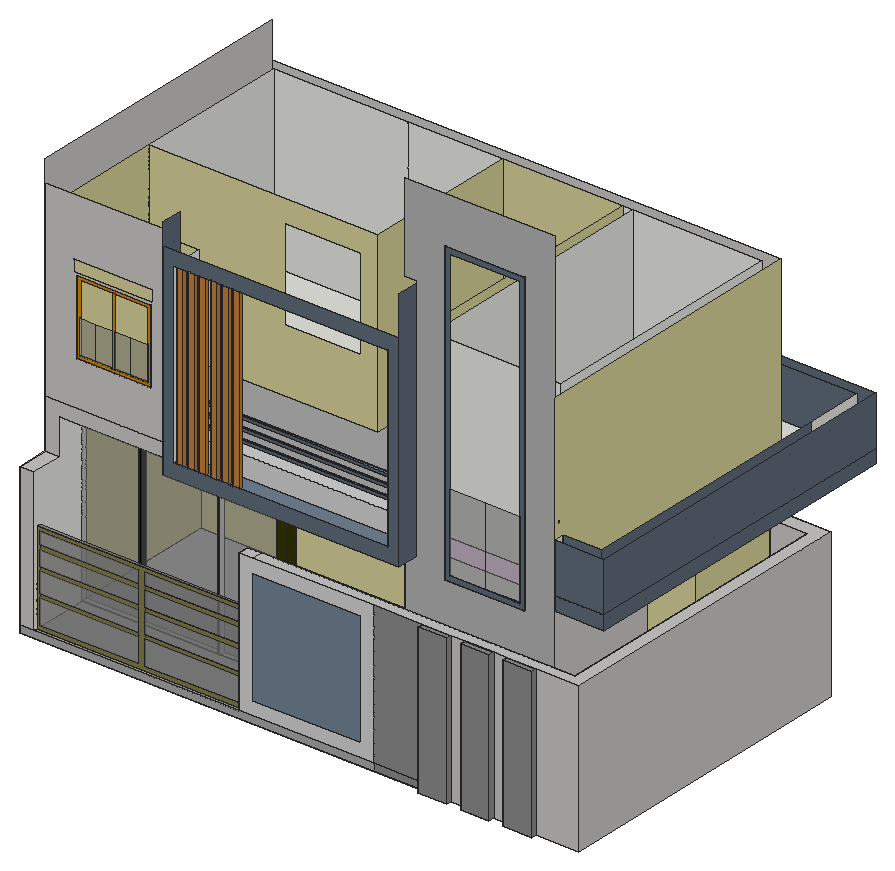
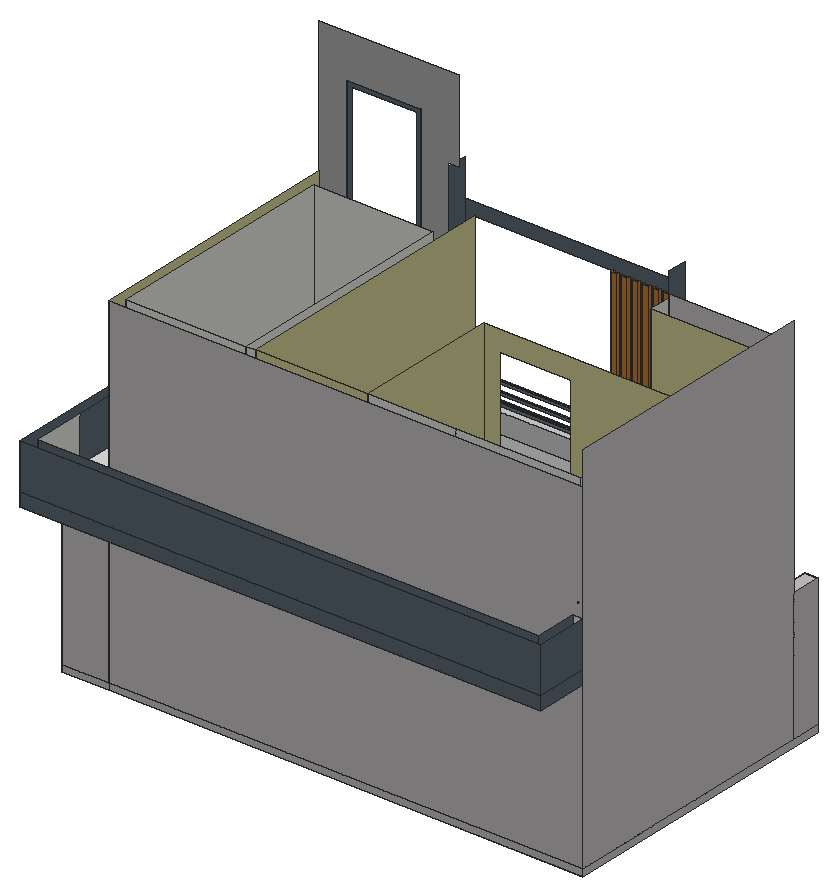
# SketchUp Ruby script. Lengths in inches.
U = 1.inch
M = Sketchup.active_model
def pt(a) = Geom::Point3d.new(a.map { |v| v * U })
def face(e, loops, mat)
  f = e.add_face(loops[0].map { |a| pt(a) })
  loops[1..].each { |l| e.add_face(l.map { |a| pt(a) }).erase! }
  f.material = f.back_material = mat if mat
  f
end
# faces: each face lists its corners as indices into pts; further lists are holes
def faces(e, pts, list, mat = nil) = list.each { |f| face(e, (f[0].is_a?(Array) ? f : [f]).map { |l| l.map { |i| pts[i] } }, mat) }
# xy, xz, yz: faces in a plane at the given z, y or x. An outline is a flat list of corners, or four numbers for a rectangle; further outlines are holes
def ring(l) = l.size == 4 ? [[l[0], l[1]], [l[2], l[1]], [l[2], l[3]], [l[0], l[3]]] : l.each_slice(2).to_a
def flat(e, list, mat, &to3) = list.each { |f| face(e, (f[0].is_a?(Array) ? f : [f]).map { |l| ring(l).map { |u, v| to3.(u, v) } }, mat) }
def xy(e, z, list, mat = nil) = flat(e, list, mat) { |x, y| [x, y, z] }
def xz(e, y, list, mat = nil) = flat(e, list, mat) { |x, z| [x, y, z] }
def yz(e, x, list, mat = nil) = flat(e, list, mat) { |y, z| [x, y, z] }
def lines(e, pts, list) = list.each { |a, b| e.add_line(pt(pts[a]), pt(pts[b])) }
# prism: a flat outline (further loops are holes) pulled along v
def prism(e, loops, v, mat = nil)
  f = face(e, loops, mat); d = Geom::Vector3d.new(v.map { |x| x * U })
  f.pushpull(f.normal.samedirection?(d) ? d.length : -d.length)
end
def box(e, o, s, mat = nil) = prism(e, [[o, [o[0] + s[0], o[1], o[2]], [o[0] + s[0], o[1] + s[1], o[2]], [o[0], o[1] + s[1], o[2]]]], [0, 0, s[2]], mat)
def at(x, y, z, deg = 0) = Geom::Transformation.translation(pt([x, y, z])) * Geom::Transformation.rotation(ORIGIN, Z_AXIS, deg.degrees)
def axes(o, x, y, z) = Geom::Transformation.new([*x, 0, *y, 0, *z, 0, *pt(o).to_a, 1])
def part(name) = M.definitions.add(name)
# library, detail: a bought-in or finely detailed component or shape, given as its bounding box
def library(name, o, s) = part(name).tap { |d| box(d.entities, o, s) }
def detail(e, o, s) = box(e.add_group.entities, o, s)
def put(e, d, t, mat = nil) = e.add_instance(d, t).tap { |i| i.material = mat if mat }
def group(e, t, mat = nil) = e.add_group.tap { |g| g.transformation = t; g.material = mat if mat }.entities
root = M.entities
M.materials.add("[0010_Snow]").color = [198, 195, 195]
M.materials.add("[0022_Maroon]").color = [61, 0, 0]
M.materials.add("[0038_Orange]").color = [211, 136, 0]
M.materials.add("[0040_Peru]").color = [191, 124, 58]
M.materials.add("[0048_PaleGoldenrod]").color = [211, 206, 151]
M.materials.add("[0053_Ivory]").color = [255, 255, 240]
M.materials.add("[0057_DarkKhaki]").color = [127, 123, 72]
M.materials.add("[0058_Olive]").color = [53, 53, 0]
M.materials.add("[0111_SlateGray]").color = [93, 106, 119]
M.materials.add("[0111_SlateGray]1").color = [112, 128, 144]
M.materials.add("[0118_Thistle]").color = [216, 191, 216]
M.materials.add("[0137_Black]").color = [0, 0, 0]
M.materials.add("[Carrera Marble]").color = [207, 207, 207]
M.materials.add("[Checker Plate]").color = [137, 137, 137]
M.materials.add("[Cladding Siding White]").color = [173, 173, 173]
M.materials.add("[Stone Vein Gray]").color = [166, 165, 165]
M.materials.add("[Translucent Glass Gray]").color = [128, 128, 128]
M.materials["[Translucent Glass Gray]"].alpha = 0.5
M.materials.add("[Wood Bamboo]").color = [177, 105, 43]
xy(root,0,[[0,9,720,543],[720,9,864,543],[864,9,948,543]])
xy(root,0,[[682.81,0,731.3,9],[754.81,0,803.3,9],[826.81,0,875.3,9]],"[Checker Plate]")
xy(root,12,[[0,9,24,63],[0,63,0,543,720,543,720,363,24,363,24,63],[609.8125,63,621.8125,89.6875],[621.8125,63,840,89.6875],[840,63,840,246,621.8125,246,621.8125,258,864,258,864,63],
  [24,111,120,120],[120,111,125,120],[125,111,254,120],[254,111,258,120],[258,111,354,120],
  [354,111,372,129],[720,363,864,543]])
xy(root,12,[[24,14.58,372,20.76]],"[0053_Ivory]")
xy(root,12,[[24,9,372,14.58],[[24,20.76,372,20.76,372,27,927,27,927,519,864,519,864,363,372,363,372,111,24,111],[609.8125,63,609.8125,89.6875,840,89.6875,840,246,609.8125,246,609.8125,258,864,258,864,63]],[24,120,354,363],[354,129,372,363]],"[Stone Vein Gray]")
xy(root,18,[[523.22,363,633.24,364]])
xy(root,118.35,[[385.28,363,477.78,364]])
xy(root,124.5625,[[391.49,363,429.53,364],[429.53,363,433.53,364],[433.53,363,471.57,364]])
xy(root,168,[[24,14.58,372,20.76]],"[Translucent Glass Gray]")
xy(root,188.875,[[55.7,363,146.7,369]])
xy(root,229.13,[[391.49,363,429.53,364],[429.53,363,433.53,364],[433.53,363,471.57,364]])
xy(root,229.13,[[523.22,363,633.24,364]],"[0022_Maroon]")
xy(root,235.35,[[385.28,363,477.78,364]])
xy(root,252,[[0,9,24,63],[372,9,396,27],[396,9,948,9,948,543,864,543,864,519,927,519,927,27,396,27]],"[0010_Snow]")
xy(root,252,[[682.81,0,731.3,9],[754.81,0,803.3,9],[826.81,0,875.3,9]],"[Checker Plate]")
xy(root,257.6875,[[55.7,363,146.7,369]])
xy(root,295.72,[[679,62,814.18,63]])
xy(root,303.72,[[687,62,746.59,63],[746.59,62,806.18,63]])
xy(root,312,[[840,63,864,63,864,258,621.8125,258,621.8125,246,840,246],[120,111,125,120],[254,111,258,120],[258,111,354,120],[0,543,720,639]])
xy(root,312,[[864,63,864,543,720,543,720,639,948,639,948,63]],"[0048_PaleGoldenrod]")
xy(root,312,[[228,27,627.8125,63]],"[0111_SlateGray]")
xy(root,312,[[[24,63,24,111,372,111,372,129,354,129,354,120,24,120,24,363,864,363,864,63,840,63,840,89.6875,609.8125,89.6875,609.8125,63],[609.8125,246,621.8125,258]]],"[0118_Thistle]")
xy(root,312,[[24,111,120,120],[125,111,254,120]],"[0137_Black]")
xy(root,336,[[251.375,27,262.5625,31.875],[270.58,27,281.76,31.875],[289.78,27,300.96,31.875],[308.98,27,320.16,31.875],[328.18,27,339.36,31.875],
  [347.375,27,358.5625,31.875],[864,63,864,81,930,81,930,621,18,621,18,543,0,543,0,639,948,639,948,63],[864,81,930,81,930,621,18,621,18,543,864,543],[627.8125,99,846,525],[18,261,405.8125,525],
  [246,525,864,543]])
xy(root,336,[[246,27,251.375,27,251.375,31.875,262.5625,31.875,262.5625,27,270.58,27,270.58,31.875,281.76,31.875,281.76,27,289.78,27,289.78,31.875,300.96,31.875,300.96,27,308.98,27,308.98,31.875,320.16,31.875,320.16,27,328.18,27,328.18,31.875,339.36,31.875,339.36,27,347.375,27,347.375,31.875,358.5625,31.875,358.5625,27,609.8125,27,609.8125,54,246,54]],"[0111_SlateGray]1")
xy(root,336,[[18,81,609.8125,81,609.8125,525,405.8125,525,405.8125,261,18,261]],"[Stone Vein Gray]")
xy(root,342,[[450.63,525,550.69,526]])
xy(root,372,[[246,54,609.8125,81]],"[Carrera Marble]")
xy(root,376.49,[[246,69.75,609.8125,74.25]])
xy(root,380.99,[[246,69.75,609.8125,74.25]],"[0111_SlateGray]1")
xy(root,394.49,[[246,69.75,609.8125,74.25]])
xy(root,398.99,[[246,69.75,609.8125,74.25]],"[0111_SlateGray]1")
xy(root,411.1875,[[52.65,63,179.28,64]],"[0137_Black]")
xy(root,412.49,[[246,69.75,609.8125,74.25]])
xy(root,416.99,[[246,69.75,609.8125,74.25]],"[0111_SlateGray]1")
xy(root,417.1875,[[58.65,63,86.31,64],[86.31,63,113.97,64],[113.97,63,117.97,64],[117.97,63,145.62,64],[145.62,63,173.28,64]])
xz(root,0,[[682.81,0,731.3,252],[754.81,0,803.3,252],[826.81,0,875.3,252]],"[Checker Plate]")
xz(root,9,[[682.81,0,731.3,252],[754.81,0,803.3,252],[826.81,0,875.3,252]])
xz(root,9,[[731.3,0,754.81,252],[803.3,0,826.81,252],[875.3,0,948,252],[0,12,24,252]],"[0010_Snow]")
xz(root,9,[[395.72,35.72,576.28,228.28]],"[0111_SlateGray]1")
xz(root,9,[[[372,12,600,252],[395.72,35.72,576.28,228.28]]],"[Carrera Marble]")
xz(root,9,[[600,0,682.81,12],[600,12,682.81,252]],"[Checker Plate]")
xz(root,9,[[0,0,600,12]],"[Stone Vein Gray]")
xz(root,14.58,[[372,60.15,376.69,66.78]],"[0053_Ivory]")
xz(root,14.58,[[[24,12,372,168],[29.375,18.65,198,162.21],[208.07,18.65,366.26,162.21]],[29.375,60.15,198,66.78],[208.07,60.15,366.26,66.78],[29.375,101.64,198,108.27],[208.07,101.64,366.26,108.27],
  [29.375,133.95,198,140.58],[208.07,135.24,366.26,141.87]],"[0057_DarkKhaki]")
xz(root,14.58,[[29.375,18.65,198,60.15],[208.07,18.65,366.26,60.15],[29.375,66.78,198,101.64],[208.07,66.78,366.26,101.64],[29.375,108.27,198,133.95],
  [208.07,108.27,366.26,135.24],[29.375,140.58,198,162.21],[208.07,141.87,366.26,162.21]],"[Translucent Glass Gray]")
xz(root,20.76,[[24,12,372,168]],"[Translucent Glass Gray]")
xz(root,27,[[372,12,927,252]],"[0010_Snow]")
xz(root,27,[[251.375,336,262.5625,636],[270.58,336,281.76,636],[289.78,336,300.96,636],[308.98,336,320.16,636],[328.18,336,339.36,636],
  [347.375,336,358.5625,636]],"[0040_Peru]")
xz(root,27,[[[228,312,627.8125,660],[246,336,609.8125,636]]],"[0111_SlateGray]")
xz(root,31.875,[[251.375,336,262.5625,636],[270.58,336,281.76,636],[289.78,336,300.96,636],[308.98,336,320.16,636],[328.18,336,339.36,636],
  [347.375,336,358.5625,636]],"[0040_Peru]")
xz(root,54,[[246,336,609.8125,372]],"[Carrera Marble]")
xz(root,62,[[[679,295.72,814.18,801.97],[687,303.72,806.18,793.97]]],"[0111_SlateGray]")
xz(root,63,[[609.8125,312,627.8125,336]])
xz(root,63,[[0,252,24,252,24,312,228,312,228,336,0,336],[[0,336,228,660],[52.65,411.1875,179.28,537.8125],[48.05,541.86,48.05,559.67,46.05,559.67,46.05,561.17,184.17,561.17,184.17,559.67,182.67,559.67,182.67,541.86]]],"[0010_Snow]")
xz(root,63,[[113.97,417.1875,117.97,531.8125]],"[0038_Orange]")
xz(root,63,[[864,312,948,336],[864,336,948,420]],"[0111_SlateGray]")
xz(root,63,[[[609.8125,12,864,12,864,882,609.8125,882,609.8125,732,629.8125,732,629.8125,726.875,627.8125,726.875,627.8125,312,609.8125,312],[679,295.72,814.18,801.97]]],"[Cladding Siding White]")
xz(root,63,[[687,303.72,746.59,435.72],[746.59,303.72,806.18,435.72],[58.65,417.1875,86.31,474.5],[86.31,417.1875,113.97,474.5],[117.97,417.1875,145.62,474.5],
  [145.62,417.1875,173.28,474.5]],"[Translucent Glass Gray]")
xz(root,64,[[[52.65,411.1875,179.28,537.8125],[58.65,417.1875,173.28,531.8125]]],"[0038_Orange]")
xz(root,69.75,[[246,376.49,609.8125,380.99],[246,394.49,609.8125,398.99],[246,412.49,609.8125,416.99]],"[0111_SlateGray]")
xz(root,74.25,[[246,376.49,609.8125,380.99],[246,394.49,609.8125,398.99],[246,412.49,609.8125,416.99]],"[0111_SlateGray]1")
xz(root,81,[[18,336,246,636]],"[0048_PaleGoldenrod]")
xz(root,81,[[864,336,930,420]],"[0111_SlateGray]")
xz(root,81,[[246,336,609.8125,372]],"[Carrera Marble]")
xz(root,89.6875,[[609.8125,12,840,312]])
xz(root,99,[[627.8125,336,846,636]])
xz(root,111,[[354,12,372,312]],"[0058_Olive]")
xz(root,111,[[120,12,125,312],[254,12,258,312]],"[0137_Black]")
xz(root,111,[[24,12,120,312],[125,12,254,312],[258,12,354,312]],"[Translucent Glass Gray]")
xz(root,120,[[120,12,125,312],[254,12,258,312]])
xz(root,129,[[354,12,372,312]],"[0058_Olive]")
xz(root,246,[[609.8125,12,840,312]],"[0010_Snow]")
xz(root,258,[[609.8125,12,621.8125,312],[621.8125,12,840,312],[840,12,864,312]])
xz(root,261,[[[18,336,405.8125,636],[247.48,443.89,376.91,598.64]]],"[0048_PaleGoldenrod]")
xz(root,363,[[[517.22,12,639.24,235.13],[523.22,18,633.24,229.13]],[429.53,124.5625,433.53,229.13]],"[0022_Maroon]")
xz(root,363,[[[24,12,517.22,12,517.22,235.13,639.24,235.13,639.24,12,864,12,864,312,24,312],[385.28,118.35,477.78,235.35],[55.7,188.875,146.7,257.6875]]],"[0048_PaleGoldenrod]")
xz(root,363,[[391.49,124.5625,429.53,229.13],[433.53,124.5625,471.57,229.13]],"[Translucent Glass Gray]")
xz(root,364,[[[385.28,118.35,477.78,235.35],[391.49,124.5625,471.57,229.13]]],"[0022_Maroon]")
xz(root,364,[[523.22,18,633.24,229.13]],"[Wood Bamboo]")
xz(root,369,[[55.7,188.875,146.7,257.6875]],"[Translucent Glass Gray]")
xz(root,519,[[864,12,927,252]],"[0010_Snow]")
xz(root,525,[[18,336,246,636],[246,336,405.8125,636],[609.8125,336,627.8125,636],[627.8125,336,846,636]])
xz(root,525,[[[444.63,336,556.69,535.0625],[450.63,342,550.69,529.0625]]],"[0022_Maroon]")
xz(root,525,[[405.8125,336,444.63,336,444.63,535.0625,556.69,535.0625,556.69,336,609.8125,336,609.8125,636,405.8125,636]],"[0048_PaleGoldenrod]")
xz(root,526,[[450.63,342,550.69,529.0625]],"[Wood Bamboo]")
xz(root,543,[[0,312,864,336],[0,336,18,420]])
xz(root,543,[[0,0,864,12],[864,0,948,12],[0,12,864,312],[864,12,948,252],[[18,336,18,420,0,420,0,636,864,636,864,336],[9,441,9.78,441.1,10.5,441.4,11.12,441.88,11.6,442.5,11.9,443.22,12,444,11.9,444.78,11.6,445.5,11.12,446.12,10.5,446.6,9.78,446.9,9,447,8.22,446.9,7.5,446.6,6.88,446.12,6.4,445.5,6.1,444.78,6,444,6.1,443.22,6.4,442.5,6.88,441.88,7.5,441.4,8.22,441.1]]],"[0010_Snow]")
xz(root,621,[[18,336,930,420]],"[0111_SlateGray]")
xz(root,639,[[0,312,948,336],[0,336,948,420]],"[0111_SlateGray]")
yz(root,0,[[9,0,543,12],[9,12,63,252],[63,12,543,696]],"[0010_Snow]")
yz(root,0,[[543,312,639,336],[543,336,639,420]],"[0111_SlateGray]")
yz(root,18,[[261,336,525,636]])
yz(root,18,[[81,336,261,636]],"[0048_PaleGoldenrod]")
yz(root,18,[[543,336,621,420]],"[0111_SlateGray]")
yz(root,24,[[9,12,14.58,12,14.58,168,20.76,168,20.76,12,111,12,111,312,63,312,63,252,9,252],[111,12,120,312]])
yz(root,24,[[120,12,363,312]],"[0048_PaleGoldenrod]")
yz(root,24,[[14.58,12,20.76,168]],"[0053_Ivory]")
yz(root,52.65,[[63,411.1875,64,537.8125]],"[0137_Black]")
yz(root,55.7,[[363,188.875,369,257.6875]])
yz(root,58.65,[[63,417.1875,64,474.5]])
yz(root,120,[[111,12,120,312]],"[0137_Black]")
yz(root,125,[[111,12,120,312]],"[0137_Black]")
yz(root,146.7,[[363,188.875,369,257.6875]])
yz(root,173.28,[[63,417.1875,64,474.5]])
yz(root,179.28,[[63,411.1875,64,537.8125]],"[0137_Black]")
yz(root,228,[[27,312,63,696]],"[0111_SlateGray]")
yz(root,246,[[[27,336,54,336,54,372,81,372,81,636,27,636],[69.75,376.49,74.25,380.99],[69.75,412.49,74.25,416.99],[69.75,394.49,74.25,398.99]],[54,336,81,372],[69.75,376.49,74.25,380.99],[69.75,412.49,74.25,416.99]])
yz(root,251.375,[[27,336,31.875,636]],"[0040_Peru]")
yz(root,254,[[111,12,120,312]],"[0137_Black]")
yz(root,258,[[111,12,120,312]])
yz(root,262.5625,[[27,336,31.875,636]],"[0040_Peru]")
yz(root,270.58,[[27,336,31.875,636]],"[0040_Peru]")
yz(root,281.76,[[27,336,31.875,636]],"[0040_Peru]")
yz(root,289.78,[[27,336,31.875,636]],"[0040_Peru]")
yz(root,300.96,[[27,336,31.875,636]],"[0040_Peru]")
yz(root,308.98,[[27,336,31.875,636]],"[0040_Peru]")
yz(root,320.16,[[27,336,31.875,636]],"[0040_Peru]")
yz(root,328.18,[[27,336,31.875,636]],"[0040_Peru]")
yz(root,339.36,[[27,336,31.875,636]],"[0040_Peru]")
yz(root,347.375,[[27,336,31.875,636]],"[0040_Peru]")
yz(root,354,[[111,12,129,312]],"[0058_Olive]")
yz(root,358.5625,[[27,336,31.875,636]],"[0040_Peru]")
yz(root,372,[[9,12,9,252,27,252,27,12,20.76,12,20.76,168,14.58,168,14.58,12]],"[0010_Snow]")
yz(root,372,[[14.58,12,20.76,168]],"[0053_Ivory]")
yz(root,372,[[111,12,129,312]],"[0058_Olive]")
yz(root,385.28,[[363,118.35,364,235.35]])
yz(root,391.49,[[363,124.5625,364,229.13]])
yz(root,405.8125,[[261,336,525,636]],"[0048_PaleGoldenrod]")
yz(root,450.63,[[525,342,526,529.0625]])
yz(root,471.57,[[363,124.5625,364,229.13]])
yz(root,477.78,[[363,118.35,364,235.35]])
yz(root,523.22,[[363,18,364,229.13]],"[0022_Maroon]")
yz(root,550.69,[[525,342,526,529.0625]])
yz(root,609.8125,[[63,336,81,372]])
yz(root,609.8125,[[63,12,89.6875,312],[246,12,258,312]],"[0010_Snow]")
yz(root,609.8125,[[[27,336,27,636,525,636,525,336,81,336,81,372,54,372,54,336],[69.75,412.49,74.25,416.99],[69.75,394.49,74.25,398.99],[69.75,376.49,74.25,380.99]]],"[0048_PaleGoldenrod]")
yz(root,627.8125,[[99,336,525,636]])
yz(root,627.8125,[[27,312,63,726.875]],"[0111_SlateGray]")
yz(root,633.24,[[363,18,364,229.13]],"[0022_Maroon]")
yz(root,679,[[62,295.72,63,312],[62,312,63,801.97]])
yz(root,682.81,[[0,0,9,12]])
yz(root,682.81,[[0,12,9,252]],"[Checker Plate]")
yz(root,687,[[62,303.72,63,312],[62,312,63,435.72]])
yz(root,731.3,[[0,0,9,252]],"[Checker Plate]")
yz(root,754.81,[[0,0,9,12]])
yz(root,754.81,[[0,12,9,252]],"[Checker Plate]")
yz(root,803.3,[[0,0,9,252]],"[Checker Plate]")
yz(root,806.18,[[62,303.72,63,312],[62,312,63,435.72]])
yz(root,814.18,[[62,295.72,63,312],[62,312,63,801.97]])
yz(root,826.81,[[0,0,9,12]])
yz(root,826.81,[[0,12,9,252]],"[Checker Plate]")
yz(root,840,[[89.6875,12,246,312]],"[0010_Snow]")
yz(root,846,[[99,336,525,636]])
yz(root,864,[[519,12,543,252],[63,312,543,336],[63,336,81,420]])
yz(root,864,[[63,12,258,312]],"[0010_Snow]")
yz(root,864,[[363,12,519,12,519,252,543,252,543,312,363,312],[[81,336,543,336,543,636,63,636,63,420,81,420],[72,441,71.22,441.1,70.5,441.4,69.88,441.88,69.4,442.5,69.1,443.22,69,444,69.1,444.78,69.4,445.5,69.88,446.12,70.5,446.6,71.22,446.9,72,447,72.78,446.9,73.5,446.6,74.12,446.12,74.6,445.5,74.9,444.78,75,444,74.9,443.22,74.6,442.5,74.12,441.88,73.5,441.4,72.78,441.1]]],"[0048_PaleGoldenrod]")
yz(root,875.3,[[0,0,9,252]],"[Checker Plate]")
yz(root,927,[[27,12,519,252]],"[0010_Snow]")
yz(root,930,[[525,336,621,420]])
yz(root,930,[[81,336,525,420]],"[0111_SlateGray]")
yz(root,948,[[9,0,543,252]],"[0010_Snow]")
yz(root,948,[[63,312,639,336],[63,336,639,420]],"[0111_SlateGray]")
p = [[246,72,414.74],[609.8125,72,414.74],[609.8125,72,396.74],[609.8125,72,398.99],[246,72,396.74],[609.8125,72,378.74],
  [609.8125,72,380.99],[246,72,378.74],[609.8125,72,412.49],[609.8125,72,394.49],[609.8125,72,376.49],[376.69,14.58,108.27],
  [376.69,14.58,101.64],[372,14.58,108.27],[372,14.58,101.64],[376.69,14.58,141.87],[376.69,14.58,135.24],[372,14.58,141.87],
  [372,14.58,135.24]]
lines(root,p,[[0,1],[2,3],[4,2],[5,6],[7,5],[8,1],[9,2],[10,5],[11,12],[11,13],[14,12],[15,16],
  [15,17],[18,16]])
